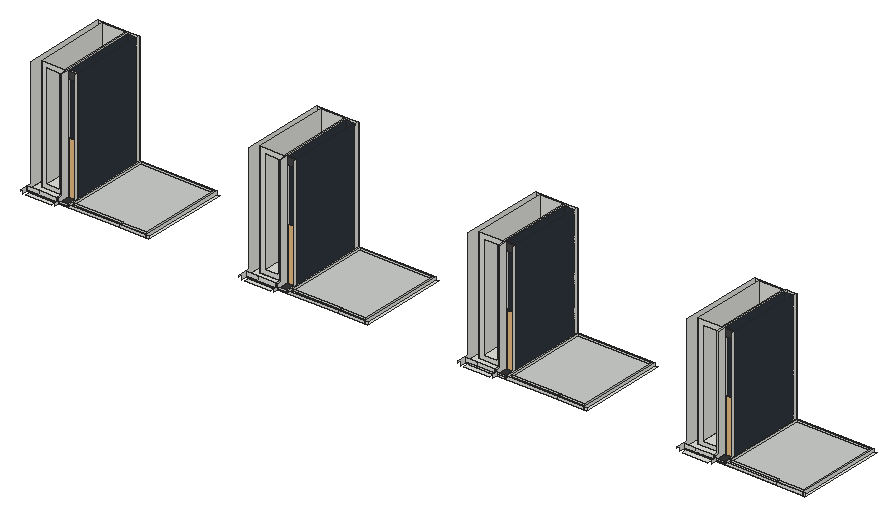
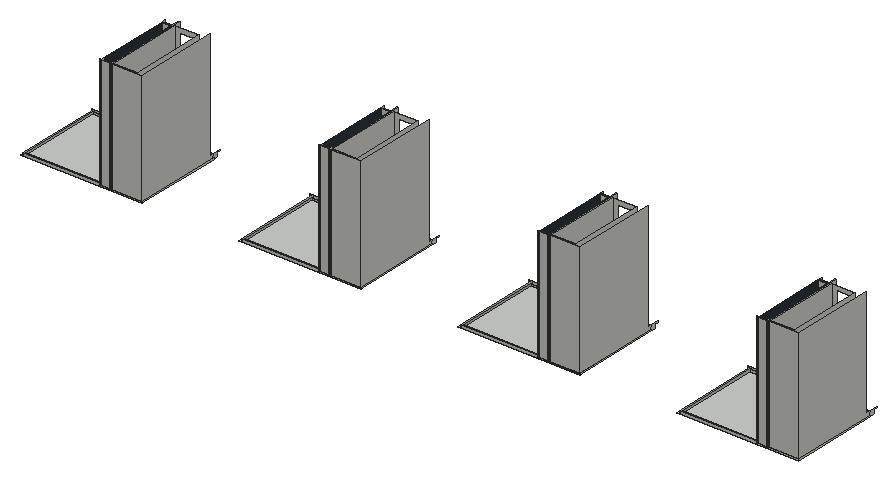
# SketchUp Ruby script. Lengths in inches.
U = 1.inch
M = Sketchup.active_model
def pt(a) = Geom::Point3d.new(a.map { |v| v * U })
def face(e, loops, mat)
  f = e.add_face(loops[0].map { |a| pt(a) })
  loops[1..].each { |l| e.add_face(l.map { |a| pt(a) }).erase! }
  f.material = f.back_material = mat if mat
  f
end
# faces: each face lists its corners as indices into pts; further lists are holes
def faces(e, pts, list, mat = nil) = list.each { |f| face(e, (f[0].is_a?(Array) ? f : [f]).map { |l| l.map { |i| pts[i] } }, mat) }
# xy, xz, yz: faces in a plane at the given z, y or x. An outline is a flat list of corners, or four numbers for a rectangle; further outlines are holes
def ring(l) = l.size == 4 ? [[l[0], l[1]], [l[2], l[1]], [l[2], l[3]], [l[0], l[3]]] : l.each_slice(2).to_a
def flat(e, list, mat, &to3) = list.each { |f| face(e, (f[0].is_a?(Array) ? f : [f]).map { |l| ring(l).map { |u, v| to3.(u, v) } }, mat) }
def xy(e, z, list, mat = nil) = flat(e, list, mat) { |x, y| [x, y, z] }
def xz(e, y, list, mat = nil) = flat(e, list, mat) { |x, z| [x, y, z] }
def yz(e, x, list, mat = nil) = flat(e, list, mat) { |y, z| [x, y, z] }
def lines(e, pts, list) = list.each { |a, b| e.add_line(pt(pts[a]), pt(pts[b])) }
# prism: a flat outline (further loops are holes) pulled along v
def prism(e, loops, v, mat = nil)
  f = face(e, loops, mat); d = Geom::Vector3d.new(v.map { |x| x * U })
  f.pushpull(f.normal.samedirection?(d) ? d.length : -d.length)
end
def box(e, o, s, mat = nil) = prism(e, [[o, [o[0] + s[0], o[1], o[2]], [o[0] + s[0], o[1] + s[1], o[2]], [o[0], o[1] + s[1], o[2]]]], [0, 0, s[2]], mat)
def at(x, y, z, deg = 0) = Geom::Transformation.translation(pt([x, y, z])) * Geom::Transformation.rotation(ORIGIN, Z_AXIS, deg.degrees)
def axes(o, x, y, z) = Geom::Transformation.new([*x, 0, *y, 0, *z, 0, *pt(o).to_a, 1])
def part(name) = M.definitions.add(name)
# library, detail: a bought-in or finely detailed component or shape, given as its bounding box
def library(name, o, s) = part(name).tap { |d| box(d.entities, o, s) }
def detail(e, o, s) = box(e.add_group.entities, o, s)
def put(e, d, t, mat = nil) = e.add_instance(d, t).tap { |i| i.material = mat if mat }
def group(e, t, mat = nil) = e.add_group.tap { |g| g.transformation = t; g.material = mat if mat }.entities
root = M.entities
M.materials.add("[Basic Tile]").color = [203, 206, 202]
M.materials.add("[Granite Dark Gray]").color = [69, 68, 68]
M.materials.add("[Mosaic Hexagonal Tile]").color = [48, 55, 63]
M.materials.add("[Slate Light Tile]").color = [54, 54, 54]
c1 = library("Scandinavian Door w/ Glass Wall\#2",[-41.94,78.85,0],[6.47,62.99,82.68])
xy(root,132,[[327.6,559.875,474.41,586.25],[1578.23,559.875,1725.04,586.25],[2828.85,559.875,2975.66,586.25],[4079.48,559.875,4226.29,586.25],[308.62,589.17,310,1096.5],
  [310,589.17,310,1096.5,990.19,1096.5,990.19,589.17,835.39,589.17,835.39,1088.45,376.61,1088.45,376.61,589.17],[376.61,589.17,835.39,1088.45],[990.19,589.17,1005.5,1096.5],[1559.25,589.17,1560.62,1096.5],[1560.62,589.17,1560.62,1096.5,2240.81,1096.5,2240.81,589.17,2086.01,589.17,2086.01,1088.45,1627.23,1088.45,1627.23,589.17],
  [1627.23,589.17,2086.01,1088.45],[2240.81,589.17,2256.12,1096.5],[2809.87,589.17,2811.25,1096.5],[2811.25,589.17,2811.25,1096.5,3491.44,1096.5,3491.44,589.17,3336.64,589.17,3336.64,1088.45,2877.86,1088.45,2877.86,589.17],[2877.86,589.17,3336.64,1088.45],
  [3491.44,589.17,3506.75,1096.5],[4060.5,589.17,4061.87,1096.5],[4061.87,589.17,4061.87,1096.5,4742.06,1096.5,4742.06,589.17,4587.26,589.17,4587.26,1088.45,4128.48,1088.45,4128.48,589.17],[4128.48,589.17,4587.26,1088.45],[4742.06,589.17,4757.37,1096.5]])
xy(root,138,[[308.62,589.17,310,1096.5],[[310,589.17,482.97,1096.5],[341.26,653.8,475.14,1088.67]],[482.97,589.17,492.21,1096.5],[543.03,589.17,551.76,1096.5],[1559.25,589.17,1560.62,1096.5],
  [[1560.62,589.17,1733.59,1096.5],[1591.89,653.8,1725.77,1088.67]],[1733.59,589.17,1742.84,1096.5],[1793.65,589.17,1802.38,1096.5],[2809.87,589.17,2811.25,1096.5],[[2811.25,589.17,2984.22,1096.5],[2842.51,653.8,2976.39,1088.67]],
  [2984.22,589.17,2993.46,1096.5],[3044.28,589.17,3053.01,1096.5],[4060.5,589.17,4061.87,1096.5],[[4061.87,589.17,4234.84,1096.5],[4093.14,653.8,4227.02,1088.67]],[4234.84,589.17,4244.09,1096.5],
  [4294.9,589.17,4303.63,1096.5],[341.26,653.8,475.14,1088.67],[1591.89,653.8,1725.77,1088.67],[2842.51,653.8,2976.39,1088.67],[4093.14,653.8,4227.02,1088.67],
  [492.21,656.57,496.1,665.86],[535.93,656.57,543.03,665.86],[1742.84,656.57,1746.73,665.86],[1786.56,656.57,1793.65,665.86],[2993.46,656.57,2997.35,665.86],
  [3037.18,656.57,3044.28,665.86],[4244.09,656.57,4247.98,665.86],[4287.81,656.57,4294.9,665.86],[492.21,665.86,543.03,1079.1875],[1742.84,665.86,1793.65,1079.1875],
  [2993.46,665.86,3044.28,1079.1875],[4244.09,665.86,4294.9,1079.1875],[492.21,1079.1875,543.03,1096.5],[1742.84,1079.1875,1793.65,1096.5],[2993.46,1079.1875,3044.28,1096.5],
  [4244.09,1079.1875,4294.9,1096.5]])
xy(root,138,[[835.39,608.75,979.42,608.75,979.42,1090.24,558.02,1090.24,558.02,616,835.39,616],[2086.01,608.75,2230.05,608.75,2230.05,1090.24,1808.65,1090.24,1808.65,616,2086.01,616],[3336.64,608.75,3480.67,608.75,3480.67,1090.24,3059.27,1090.24,3059.27,616,3336.64,616],[4587.26,608.75,4731.3,608.75,4731.3,1090.24,4309.9,1090.24,4309.9,616,4587.26,616]],"[Basic Tile]")
xy(root,138,[[492.21,589.17,543.03,589.17,543.03,656.57,535.93,656.57,535.93,665.86,496.1,665.86,496.1,656.57,492.21,656.57],[1742.84,589.17,1793.65,589.17,1793.65,656.57,1786.56,656.57,1786.56,665.86,1746.73,665.86,1746.73,656.57,1742.84,656.57],[2993.46,589.17,3044.28,589.17,3044.28,656.57,3037.18,656.57,3037.18,665.86,2997.35,665.86,2997.35,656.57,2993.46,656.57],[4244.09,589.17,4294.9,589.17,4294.9,656.57,4287.81,656.57,4287.81,665.86,4247.98,665.86,4247.98,656.57,4244.09,656.57]],"[Slate Light Tile]")
xz(root,589.17,[[308.62,132,310,138],[310,132,376.61,138],[376.61,132,492.21,138],[492.21,132,835.39,132,835.39,148.4375,551.76,148.4375,551.76,138,492.21,138],[835.39,132,990.19,148.4375],
  [990.19,132,1005.5,148.4375],[1559.25,132,1560.62,138],[1560.62,132,1627.23,138],[1627.23,132,1742.84,138],[1742.84,132,2086.01,132,2086.01,148.4375,1802.38,148.4375,1802.38,138,1742.84,138],
  [2086.01,132,2240.81,148.4375],[2240.81,132,2256.12,148.4375],[2809.87,132,2811.25,138],[2811.25,132,2877.86,138],[2877.86,132,2993.46,138],
  [2993.46,132,3336.64,132,3336.64,148.4375,3053.01,148.4375,3053.01,138,2993.46,138],[3336.64,132,3491.44,148.4375],[3491.44,132,3506.75,148.4375],[4060.5,132,4061.87,138],[4061.87,132,4128.48,138],
  [4128.48,132,4244.09,138],[4244.09,132,4587.26,132,4587.26,148.4375,4303.63,148.4375,4303.63,138,4244.09,138],[4587.26,132,4742.06,148.4375],[4742.06,132,4757.37,148.4375],[310,138,376.61,161.375],
  [376.61,138,482.97,161.375],[482.97,138,492.21,161.375],[492.21,138,543.03,148.4375],[543.03,138,551.76,148.4375],[1560.62,138,1627.23,161.375],
  [1627.23,138,1733.59,161.375],[1733.59,138,1742.84,161.375],[1742.84,138,1793.65,148.4375],[1793.65,138,1802.38,148.4375],[2811.25,138,2877.86,161.375],
  [2877.86,138,2984.22,161.375],[2984.22,138,2993.46,161.375],[2993.46,138,3044.28,148.4375],[3044.28,138,3053.01,148.4375],[4061.87,138,4128.48,161.375],
  [4128.48,138,4234.84,161.375],[4234.84,138,4244.09,161.375],[4244.09,138,4294.9,148.4375],[4294.9,138,4303.63,148.4375]])
xz(root,608.75,[[835.39,138,979.42,148.4375],[2086.01,138,2230.05,148.4375],[3336.64,138,3480.67,148.4375],[4587.26,138,4731.3,148.4375]])
xz(root,616,[[558.02,138,835.39,148.4375],[1808.65,138,2086.01,148.4375],[3059.27,138,3336.64,148.4375],[4309.9,138,4587.26,148.4375]])
xz(root,653.8,[[[341.26,138,475.14,784.4375],[367.98,161.375,449.07,759.44]],[[1591.89,138,1725.77,784.4375],[1618.6,161.375,1699.7,759.44]],[[2842.51,138,2976.39,784.4375],[2869.23,161.375,2950.32,759.44]],[[4093.14,138,4227.02,784.4375],[4119.85,161.375,4200.95,759.44]]])
xz(root,656.57,[[492.21,138,496.1,138,496.1,742.22,535.93,742.22,535.93,138,543.03,138,543.03,784.4375,492.21,784.4375],[1742.84,138,1746.73,138,1746.73,742.22,1786.56,742.22,1786.56,138,1793.65,138,1793.65,784.4375,1742.84,784.4375],[2993.46,138,2997.35,138,2997.35,742.22,3037.18,742.22,3037.18,138,3044.28,138,3044.28,784.4375,2993.46,784.4375],[4244.09,138,4247.98,138,4247.98,742.22,4287.81,742.22,4287.81,138,4294.9,138,4294.9,784.4375,4244.09,784.4375]],"[Granite Dark Gray]")
xz(root,665.86,[[492.21,138,492.21,784.4375,543.03,784.4375,543.03,138,535.93,138,535.93,742.22,496.1,742.22,496.1,138],[1742.84,138,1742.84,784.4375,1793.65,784.4375,1793.65,138,1786.56,138,1786.56,742.22,1746.73,742.22,1746.73,138],[2993.46,138,2993.46,784.4375,3044.28,784.4375,3044.28,138,3037.18,138,3037.18,742.22,2997.35,742.22,2997.35,138],[4244.09,138,4244.09,784.4375,4294.9,784.4375,4294.9,138,4287.81,138,4287.81,742.22,4247.98,742.22,4247.98,138]])
xz(root,1079.1875,[[492.21,138,543.03,784.4375],[1742.84,138,1793.65,784.4375],[2993.46,138,3044.28,784.4375],[4244.09,138,4294.9,784.4375]],"[Mosaic Hexagonal Tile]")
xz(root,1088.67,[[341.26,138,475.14,784.4375],[1591.89,138,1725.77,784.4375],[2842.51,138,2976.39,784.4375],[4093.14,138,4227.02,784.4375]])
xz(root,1090.24,[[558.02,138,979.42,148.4375],[1808.65,138,2230.05,148.4375],[3059.27,138,3480.67,148.4375],[4309.9,138,4731.3,148.4375]])
xz(root,1096.5,[[308.62,132,308.62,138,551.76,138,551.76,148.4375,990.19,148.4375,990.19,132],[1559.25,132,1559.25,138,1802.38,138,1802.38,148.4375,2240.81,148.4375,2240.81,132],[2809.87,132,2809.87,138,3053.01,138,3053.01,148.4375,3491.44,148.4375,3491.44,132],[4060.5,132,4060.5,138,4303.63,138,4303.63,148.4375,4742.06,148.4375,4742.06,132],[310,138,482.97,784.4375],
  [482.97,138,492.21,784.4375],[492.21,138,543.03,784.4375],[543.03,138,551.76,784.4375],[1560.62,138,1733.59,784.4375],[1733.59,138,1742.84,784.4375],
  [1742.84,138,1793.65,784.4375],[1793.65,138,1802.38,784.4375],[2811.25,138,2984.22,784.4375],[2984.22,138,2993.46,784.4375],[2993.46,138,3044.28,784.4375],
  [3044.28,138,3053.01,784.4375],[4061.87,138,4234.84,784.4375],[4234.84,138,4244.09,784.4375],[4244.09,138,4294.9,784.4375],[4294.9,138,4303.63,784.4375]])
yz(root,308.62,[[589.17,132,1096.5,138]])
yz(root,310,[[559.875,132,559.875,155.3125,542.125,155.3125,542.125,161.375,589.17,161.375,589.17,132],[589.17,138,589.17,161.375,613.74,161.375,613.74,784.4375,1096.5,784.4375,1096.5,138]])
yz(root,341.26,[[653.8,138,1088.67,784.4375]])
yz(root,475.14,[[653.8,138,1088.67,784.4375]])
yz(root,482.97,[[589.17,138,1096.5,138,1096.5,784.4375,613.74,784.4375,613.74,161.375,589.17,161.375]])
yz(root,492.21,[[559.875,132,589.17,148.4375],[589.17,138,656.57,138,656.57,784.4375,613.74,784.4375,613.74,161.375,589.17,161.375],[1079.1875,138,1096.5,784.4375]])
yz(root,492.21,[[665.86,138,1079.1875,784.4375]],"[Mosaic Hexagonal Tile]")
yz(root,496.1,[[656.57,138,665.86,742.22]])
yz(root,535.93,[[656.57,138,665.86,742.22]])
yz(root,543.03,[[589.17,138,589.17,148.4375,640.11,148.4375,640.11,784.4375,656.57,784.4375,656.57,138],[1079.1875,138,1096.5,784.4375]])
yz(root,543.03,[[665.86,138,1079.1875,784.4375]],"[Mosaic Hexagonal Tile]")
yz(root,551.76,[[589.17,138,1096.5,148.4375]])
yz(root,558.02,[[616,138,1090.24,148.4375]])
yz(root,835.39,[[608.75,138,616,148.4375]])
yz(root,979.42,[[608.75,138,1090.24,148.4375]],"[Basic Tile]")
yz(root,990.19,[[589.17,132,1096.5,148.4375]])
yz(root,1559.25,[[589.17,132,1096.5,138]])
yz(root,1560.62,[[559.875,132,559.875,155.3125,542.125,155.3125,542.125,161.375,589.17,161.375,589.17,132],[589.17,138,589.17,161.375,613.74,161.375,613.74,784.4375,1096.5,784.4375,1096.5,138]])
yz(root,1591.89,[[653.8,138,1088.67,784.4375]])
yz(root,1725.77,[[653.8,138,1088.67,784.4375]])
yz(root,1733.59,[[589.17,138,1096.5,138,1096.5,784.4375,613.74,784.4375,613.74,161.375,589.17,161.375]])
yz(root,1742.84,[[559.875,132,589.17,148.4375],[589.17,138,656.57,138,656.57,784.4375,613.74,784.4375,613.74,161.375,589.17,161.375],[1079.1875,138,1096.5,784.4375]])
yz(root,1742.84,[[665.86,138,1079.1875,784.4375]],"[Mosaic Hexagonal Tile]")
yz(root,1746.73,[[656.57,138,665.86,742.22]])
yz(root,1786.56,[[656.57,138,665.86,742.22]])
yz(root,1793.65,[[589.17,138,589.17,148.4375,640.11,148.4375,640.11,784.4375,656.57,784.4375,656.57,138],[1079.1875,138,1096.5,784.4375]])
yz(root,1793.65,[[665.86,138,1079.1875,784.4375]],"[Mosaic Hexagonal Tile]")
yz(root,1802.38,[[589.17,138,1096.5,148.4375]])
yz(root,1808.65,[[616,138,1090.24,148.4375]])
yz(root,2086.01,[[608.75,138,616,148.4375]])
yz(root,2230.05,[[608.75,138,1090.24,148.4375]],"[Basic Tile]")
yz(root,2240.81,[[589.17,132,1096.5,148.4375]])
yz(root,2809.87,[[589.17,132,1096.5,138]])
yz(root,2811.25,[[559.875,132,559.875,155.3125,542.125,155.3125,542.125,161.375,589.17,161.375,589.17,132],[589.17,138,589.17,161.375,613.74,161.375,613.74,784.4375,1096.5,784.4375,1096.5,138]])
yz(root,2842.51,[[653.8,138,1088.67,784.4375]])
yz(root,2976.39,[[653.8,138,1088.67,784.4375]])
yz(root,2984.22,[[589.17,138,1096.5,138,1096.5,784.4375,613.74,784.4375,613.74,161.375,589.17,161.375]])
yz(root,2993.46,[[559.875,132,589.17,148.4375],[589.17,138,656.57,138,656.57,784.4375,613.74,784.4375,613.74,161.375,589.17,161.375],[1079.1875,138,1096.5,784.4375]])
yz(root,2993.46,[[665.86,138,1079.1875,784.4375]],"[Mosaic Hexagonal Tile]")
yz(root,2997.35,[[656.57,138,665.86,742.22]])
yz(root,3037.18,[[656.57,138,665.86,742.22]])
yz(root,3044.28,[[589.17,138,589.17,148.4375,640.11,148.4375,640.11,784.4375,656.57,784.4375,656.57,138],[1079.1875,138,1096.5,784.4375]])
yz(root,3044.28,[[665.86,138,1079.1875,784.4375]],"[Mosaic Hexagonal Tile]")
yz(root,3053.01,[[589.17,138,1096.5,148.4375]])
yz(root,3059.27,[[616,138,1090.24,148.4375]])
yz(root,3336.64,[[608.75,138,616,148.4375]])
yz(root,3480.67,[[608.75,138,1090.24,148.4375]],"[Basic Tile]")
yz(root,3491.44,[[589.17,132,1096.5,148.4375]])
yz(root,4060.5,[[589.17,132,1096.5,138]])
yz(root,4061.87,[[559.875,132,559.875,155.3125,542.125,155.3125,542.125,161.375,589.17,161.375,589.17,132],[589.17,138,589.17,161.375,613.74,161.375,613.74,784.4375,1096.5,784.4375,1096.5,138]])
yz(root,4093.14,[[653.8,138,1088.67,784.4375]])
yz(root,4227.02,[[653.8,138,1088.67,784.4375]])
yz(root,4234.84,[[589.17,138,1096.5,138,1096.5,784.4375,613.74,784.4375,613.74,161.375,589.17,161.375]])
yz(root,4244.09,[[559.875,132,589.17,148.4375],[589.17,138,656.57,138,656.57,784.4375,613.74,784.4375,613.74,161.375,589.17,161.375],[1079.1875,138,1096.5,784.4375]])
yz(root,4244.09,[[665.86,138,1079.1875,784.4375]],"[Mosaic Hexagonal Tile]")
yz(root,4247.98,[[656.57,138,665.86,742.22]])
yz(root,4287.81,[[656.57,138,665.86,742.22]])
yz(root,4294.9,[[589.17,138,589.17,148.4375,640.11,148.4375,640.11,784.4375,656.57,784.4375,656.57,138],[1079.1875,138,1096.5,784.4375]])
yz(root,4294.9,[[665.86,138,1079.1875,784.4375]],"[Mosaic Hexagonal Tile]")
yz(root,4303.63,[[589.17,138,1096.5,148.4375]])
yz(root,4309.9,[[616,138,1090.24,148.4375]])
yz(root,4587.26,[[608.75,138,616,148.4375]])
yz(root,4731.3,[[608.75,138,1090.24,148.4375]],"[Basic Tile]")
yz(root,4742.06,[[589.17,132,1096.5,148.4375]])
p = [[3415.16,880.43,131.5],[3052.36,880.43,131.5]]
lines(root,p,[[0,1]])
put(root,c1,axes([446.25,621.1,138],[0,-1,0],[0.63229,0,0],[0,0,3.65663]))
put(root,c1,axes([2947.5,621.1,138],[0,-1,0],[0.63229,0,0],[0,0,3.65663]))
put(root,c1,axes([1696.87,621.1,138],[0,-1,0],[0.63229,0,0],[0,0,3.65663]))
put(root,c1,axes([4198.12,621.1,138],[0,-1,0],[0.63229,0,0],[0,0,3.65663]))
